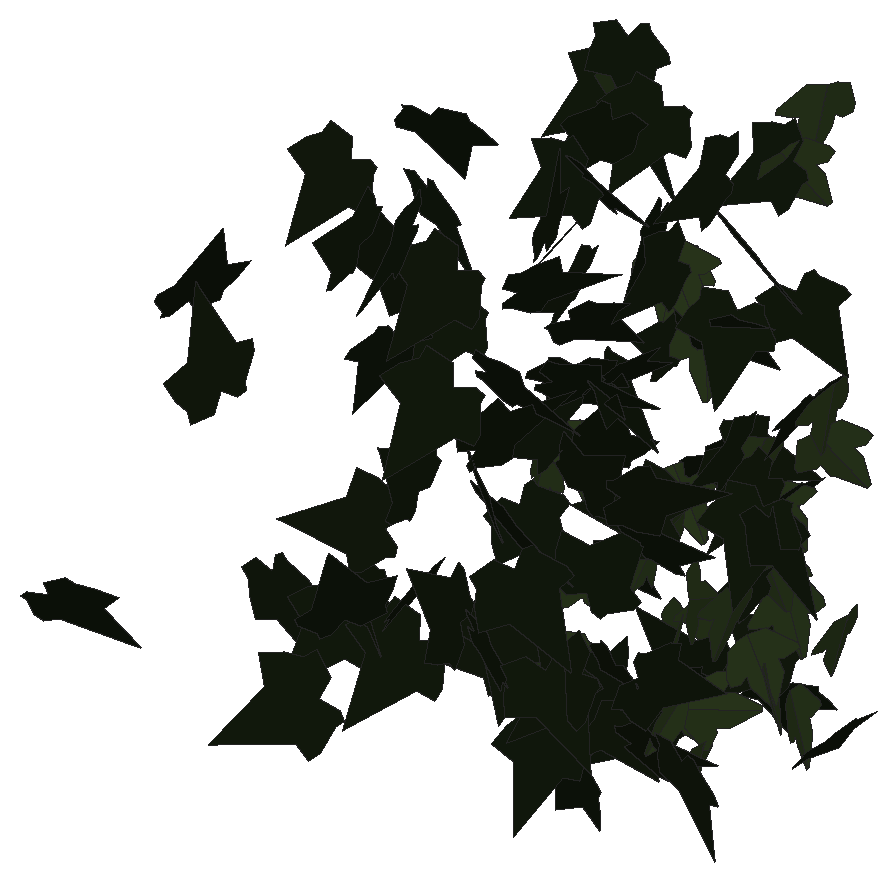
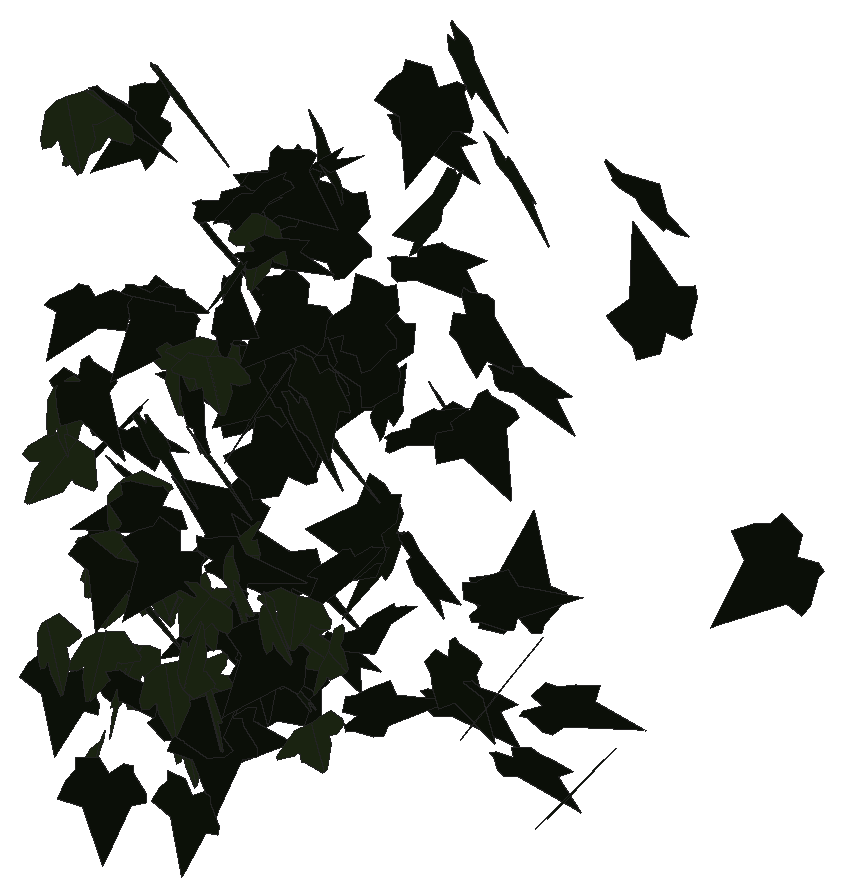
# SketchUp Ruby script. Lengths in inches.
U = 1.inch
M = Sketchup.active_model
def pt(a) = Geom::Point3d.new(a.map { |v| v * U })
def face(e, loops, mat)
  f = e.add_face(loops[0].map { |a| pt(a) })
  loops[1..].each { |l| e.add_face(l.map { |a| pt(a) }).erase! }
  f.material = f.back_material = mat if mat
  f
end
# faces: each face lists its corners as indices into pts; further lists are holes
def faces(e, pts, list, mat = nil) = list.each { |f| face(e, (f[0].is_a?(Array) ? f : [f]).map { |l| l.map { |i| pts[i] } }, mat) }
# xy, xz, yz: faces in a plane at the given z, y or x. An outline is a flat list of corners, or four numbers for a rectangle; further outlines are holes
def ring(l) = l.size == 4 ? [[l[0], l[1]], [l[2], l[1]], [l[2], l[3]], [l[0], l[3]]] : l.each_slice(2).to_a
def flat(e, list, mat, &to3) = list.each { |f| face(e, (f[0].is_a?(Array) ? f : [f]).map { |l| ring(l).map { |u, v| to3.(u, v) } }, mat) }
def xy(e, z, list, mat = nil) = flat(e, list, mat) { |x, y| [x, y, z] }
def xz(e, y, list, mat = nil) = flat(e, list, mat) { |x, z| [x, y, z] }
def yz(e, x, list, mat = nil) = flat(e, list, mat) { |y, z| [x, y, z] }
def lines(e, pts, list) = list.each { |a, b| e.add_line(pt(pts[a]), pt(pts[b])) }
# prism: a flat outline (further loops are holes) pulled along v
def prism(e, loops, v, mat = nil)
  f = face(e, loops, mat); d = Geom::Vector3d.new(v.map { |x| x * U })
  f.pushpull(f.normal.samedirection?(d) ? d.length : -d.length)
end
def box(e, o, s, mat = nil) = prism(e, [[o, [o[0] + s[0], o[1], o[2]], [o[0] + s[0], o[1] + s[1], o[2]], [o[0], o[1] + s[1], o[2]]]], [0, 0, s[2]], mat)
def at(x, y, z, deg = 0) = Geom::Transformation.translation(pt([x, y, z])) * Geom::Transformation.rotation(ORIGIN, Z_AXIS, deg.degrees)
def axes(o, x, y, z) = Geom::Transformation.new([*x, 0, *y, 0, *z, 0, *pt(o).to_a, 1])
def part(name) = M.definitions.add(name)
# library, detail: a bought-in or finely detailed component or shape, given as its bounding box
def library(name, o, s) = part(name).tap { |d| box(d.entities, o, s) }
def detail(e, o, s) = box(e.add_group.entities, o, s)
def put(e, d, t, mat = nil) = e.add_instance(d, t).tap { |i| i.material = mat if mat }
def group(e, t, mat = nil) = e.add_group.tap { |g| g.transformation = t; g.material = mat if mat }.entities
root = M.entities
M.materials.add("efeu1").color = [18, 25, 13]
M.materials.add("efeu2").color = [43, 57, 29]
c1 = part("ivyleaf_9")
p = [[1.54,2.16,1.25],[1.36,2.04,1.19],[-0.21,0.99,0.68],[-0.71,1.11,0.82],[-0.85,0.86,0.67],[-0.8,0.17,0.21],
  [-0.9,-0.01,0.1],[-0.67,-0.16,-0.02],[-0.08,-0.08,-0.05],[-0.03,-0.6,-0.4],[0.65,-0.88,-0.66],[0.83,-0.6,-0.49],
  [1.29,-0.42,-0.43],[1.8125,-0.07,-0.26],[1.21,0.44,0.15]]
faces(c1.entities,p,[[0,1,2,3,4,5,6,7,8,9,10,11,12,13,14]],"efeu1")
c2 = part("ivyleaf_10")
p = [[0,0.5,-0.03],[-0.0625,2.02,-0.43],[-0.19,2.01,-0.46],[-0.54,1.05,-0.29],[-0.52,0.625,-0.18],[-0.83,0.76,-0.28],
  [-1.16,0.64,-0.33],[-1.15,0.33,-0.24],[-0.77,-0.39,0.02],[-0.3,-0.51,0.16],[0.04,-0.48,0.23],[-0.02,2.01,-0.4375],
  [-0.06,2.01,-0.43],[0.04,-0.49,0.23],[0.67,-0.49,0.14],[1.38,0.36,-0.2],[1.375,0.51,-0.24],[0.81,0.65,-0.19],
  [0.62,0.59,-0.15],[0.6,1.09,-0.28],[0.5,1.23,-0.31]]
faces(c2.entities,p,[[0,1,2,3,4,5,6,7,8,9,10],[11,12,0,13,14,15,16,17,18,19,20]],"efeu2")
put(root,c1,axes([487.93,108.94,283.27],[1.28047,0.4773,0.27345],[0.2614,0.10282,-1.3292],[-0.52728,1.21006,0.00509]))
put(root,c1,axes([488.25,120.74,279.03],[0.66531,-1.07107,-0.28603],[-0.01199,0.30882,-1.27663],[1.19422,0.5998,0.14653]))
put(root,c1,axes([490.58,121.86,295.7],[-1.24756,-0.33673,-0.124],[0.12614,0.02537,-1.25133],[0.36459,-1.16101,0.00862]))
put(root,c1,axes([490.5,113.3,294.06],[0.7519,0.9623,0.59354],[-0.36171,-0.4621,1.23525],[1.1529,-0.77257,0.00046]))
put(root,c1,axes([491.55,120.59,278.68],[-1.20578,-0.36706,0.02195],[-0.02114,-0.00803,-1.22226],[0.39652,-1.11663,0.00157]))
put(root,c1,axes([493.79,116.03,278.13],[-1.09165,-0.45472,0.71253],[-0.6746,-0.28149,-1.15269],[0.57758,-1.18821,0.0004]))
put(root,c1,axes([494.18,119.21,283.68],[-0.63666,-0.11353,1.04614],[-1.04545,-0.27731,-0.62254],[0.31983,-1.13246,0.04757]))
put(root,c1,axes([493.28,120.4,280.03],[0.56041,-1.01215,-0.61379],[0.28817,-0.52643,1.18291],[-1.23214,-0.58348,-0.00251]))
put(root,c1,axes([495.48,118.52,295.01],[-0.3234,0.18269,-1.25426],[-1.25926,-0.40761,0.23687],[-0.38692,1.17388,0.27745]))
put(root,c1,axes([494.85,119.17,291.41],[-0.01545,0.87558,-0.83789],[0.05178,-0.80465,-0.91033],[-1.28399,-0.04299,-0.02663]))
put(root,c1,axes([495.12,120.08,281.33],[-0.61436,0.86217,-0.53743],[0.23859,-0.47202,-1.07194],[-1.05905,-0.60649,0.07027]))
put(root,c1,axes([495.47,119.46,279.48],[-1.26791,-0.58004,0.05064],[-0.04795,-0.02007,-1.36184],[0.62682,-1.17482,-0.00174]))
put(root,c1,axes([494.96,116.24,281.73],[0.81621,0.50536,0.90532],[-0.76893,-0.50108,0.94538],[0.76843,-1.03819,-0.01561]))
put(root,c1,axes([496.25,107.69,295.03],[-1.35018,0.22059,-0.35895],[-0.37798,0.00073,1.31888],[0.22987,1.29694,0.06031]))
put(root,c1,axes([495.56,121.73,291.72],[-0.62945,-0.9519,0.32133],[-0.13909,-0.28323,-1.16017],[1.07186,-0.59576,0.03815]))
put(root,c2,axes([496,126.03,283.95],[-0.05585,0.76733,-0.76603],[-0.02611,-0.7381,-0.79792],[-1.14844,-0.02054,0.0554]))
put(root,c1,axes([497.65,113.55,298.5625],[-0.71399,0.92904,0.58294],[-0.32129,0.47602,-1.18544],[-1.12693,-0.72432,-0.03136]))
put(root,c1,axes([497.79,121.96,278.97],[-0.63673,-0.23437,0.99321],[-0.89864,-0.4745,-0.65533],[0.56597,-1.01709,0.07686]))
put(root,c1,axes([498,124.14,294.07],[-0.22195,1.05914,0.2908],[-0.07545,0.27124,-1.12192],[-1.18065,-0.21644,0.01703]))
put(root,c1,axes([498.6,115.63,288.34],[-0.44952,0.70387,0.94859],[-0.52802,0.77025,-0.8502],[-1.1267,-0.6418,0.01998]))
put(root,c2,axes([498.64,126.44,284.82],[-0.33345,0.24798,1.01054],[-1.02586,0.25368,-0.38123],[-0.34727,-0.98748,0.15583]))
put(root,c2,axes([497.55,125.99,285.46],[1.05762,0.34197,0.24255],[0.23343,0.08843,-1.07869],[-0.38126,1.00277,0.01241]))
put(root,c1,axes([498.62,124.46,292.66],[-0.76152,0.84642,0.12193],[-0.0679,0.1002,-1.14559],[-0.92036,-0.70774,-0.01637]))
put(root,c1,axes([497.37,117.9,298.62],[0.82838,-0.99614,0.21737],[0.14057,-0.16356,-1.30751],[1.09023,0.77798,0.00343]))
put(root,c1,axes([499.32,116.99,282.75],[-0.77408,0.11861,-1.07409],[-1.12199,-0.03607,0.74551],[0.04086,1.2566,0.12278]))
put(root,c1,axes([498.6,116.57,302.58],[1.06494,0.63385,-0.42408],[-0.39134,-0.1901,-1.21858],[-0.71374,1.04997,0.03539]))
put(root,c1,axes([499.18,126.26,299.9],[-0.97309,-0.47861,0.43077],[-0.36109,-0.25196,-1.05916],[0.58044,-0.95912,0.06328]))
put(root,c2,axes([498.79,123.53,278.63],[0.45745,0.95813,-0.33869],[-0.12878,-0.30333,-1.0894],[-1.08531,0.43984,-0.0135]))
put(root,c1,axes([498.61,121.46,285.01],[0.27665,-0.81103,-0.82368],[-0.03201,0.8069,-0.86931],[1.22386,0.20444,0.16346]))
put(root,c2,axes([499.94,123.3,282.11],[0.43654,0.59015,-0.87113],[-0.85601,-0.39058,-0.68397],[-0.70132,0.84407,0.29258]))
put(root,c1,axes([499.2,120.26,281.35],[-0.29354,-1.2558,0.10971],[0.04408,-0.11663,-1.3346],[1.36033,-0.26721,0.06692]))
put(root,c2,axes([499.65,125.52,300.19],[-1.17327,0.17833,-0.01914],[0.01141,-0.04912,-1.14391],[-0.19328,-1.08541,0.04862]))
put(root,c1,axes([498.58,120.01,285.47],[0.96236,-0.64468,0.71352],[0.61154,-0.38769,-1.14371],[0.81229,1.05565,0.01571]))
put(root,c1,axes([499.54,124.47,282.3125],[1.08086,0.50793,0.05554],[0.04126,0.0427,-1.167],[-0.55004,1.00131,0.02159]))
put(root,c1,axes([499.7,125.96,301.93],[-0.00715,-1.08085,-0.28112],[-0.01614,0.27037,-1.12398],[1.20316,-0.0028,-0.01675]))
put(root,c1,axes([501.16,120.59,289.69],[-1.08825,0.75622,0.20973],[-0.21335,0.07236,-1.30875],[-0.81789,-1.02507,0.06234]))
put(root,c1,axes([499.99,126,299.13],[0.71012,-0.86332,-0.21957],[-0.17465,0.14202,-1.12777],[0.94384,0.67582,-0.04349]))
put(root,c2,axes([500.81,128.3,282.34],[-0.99681,0.45304,-0.10562],[-0.09466,0.05192,1.06926],[0.49241,0.92709,-0.00827]))
put(root,c1,axes([501.09,114.36,293.66],[-1.1174,-0.74824,0.09783],[-0.09095,-0.04406,-1.32784],[0.80937,-1.03797,-0.01416]))
put(root,c1,axes([501.63,126.28,290.56],[-0.6962,0.71839,0.51384],[-0.36076,0.36408,-1.00381],[-0.8698,-0.72602,0.00506]))
put(root,c1,axes([501.32,120.99,291.74],[0.48216,0.89736,-0.57571],[-0.36034,-0.45002,-1.03853],[-1.0802,0.55067,0.08946]))
put(root,c1,axes([501.34,127.53,276.62],[0.05973,1.00849,0.27515],[0.00127,0.26488,-1.05032],[-1.12602,0.05379,0.01341]))
put(root,c1,axes([501.43,111.7,301.33],[-1.07069,0.64043,-0.56187],[0.49905,-0.28027,-1.22737],[-0.75485,-1.09369,-0.01448]))
put(root,c1,axes([501.48,122.65,300.73],[-0.16617,0.42284,-1.15158],[0.11729,-1.10686,-0.45527],[-1.27472,-0.15696,0.10823]))
put(root,c1,axes([500.78,116.33,282.95],[1.11311,-0.44226,-0.57466],[-0.51259,0.29221,-1.16392],[0.56703,1.13234,0.07591]))
put(root,c1,axes([500.73,116.72,288.3],[-0.11743,-0.19889,1.22297],[0.35877,-1.13913,-0.16843],[1.23707,0.31149,0.16494]))
put(root,c1,axes([500.75,116.47,290.38],[0.41054,0.09554,1.27946],[0.993,0.83661,-0.36303],[-0.8888,0.97882,0.1854]))
put(root,c1,axes([500.34,117.6,292.59],[1.09496,-0.2857,0.58591],[0.58305,-0.16126,-1.09544],[0.35422,1.1486,-0.00806]))
put(root,c1,axes([501.75,113.72,298.82],[-1.29927,-0.40781,-0.08882],[0.09054,0.0187,-1.32104],[0.44079,-1.20591,0.00956]))
put(root,c1,axes([502.3,121.1,278.99],[-0.19234,0.78394,0.95988],[-0.66464,0.74484,-0.78146],[-1.12635,-0.57339,0.29721]))
put(root,c1,axes([501.76,120.65,299.54],[-0.62074,-0.59858,0.79763],[-0.32321,-0.73882,-0.83294],[0.99977,-0.6105,0.22595]))
put(root,c1,axes([502.66,124.33,284.79],[-0.76552,0.11117,0.89511],[-0.92454,0.09292,-0.74568],[-0.15391,-1.11111,0.0272]))
put(root,c1,axes([501.95,124.92,300.42],[-0.86795,-0.80642,0.09014],[-0.06237,-0.06482,-1.18403],[0.87373,-0.80572,0.00503]))
put(root,c1,axes([501.33,121.95,287.95],[1.12729,0.53463,0.35878],[-0.35836,-0.10816,1.21842],[0.58634,-1.09399,0.05487]))
put(root,c2,axes([501.18,126.81,284.625],[0.92731,0.25344,0.61982],[0.61929,0.16252,-0.93104],[-0.32511,1.03248,-0.00559]))
put(root,c2,axes([501.67,125.95,294.04],[1.1014,0.3935,-0.06883],[-0.05703,-0.04694,-1.13653],[-0.42716,1.02088,-0.02573]))
put(root,c1,axes([501.01,120.42,291.29],[1.04245,0.17584,0.70002],[0.69592,0.20798,-1.01749],[-0.28323,1.15822,0.07643]))
put(root,c2,axes([501.86,126.06,283.59],[-0.27404,0.07877,-1.10356],[-0.06938,-1.09002,-0.06817],[-1.14706,0.04711,0.26777]))
put(root,c1,axes([502.21,124.88,278.04],[0.47069,0.90796,-0.34427],[-0.21132,-0.27271,-1.04584],[-1.02212,0.4745,0.05769]))
put(root,c1,axes([501.86,124.9,296.1],[-0.37104,0.20867,-1.1142],[0.85439,-0.72621,-0.41094],[-0.81214,-0.85932,0.07672]))
put(root,c2,axes([502.09,125.56,279.9375],[0.73965,-0.77122,-0.18777],[-0.10942,0.15143,-1.07237],[0.84841,0.69188,0.0254]))
put(root,c2,axes([502.15,124.03,283.66],[0.87236,-0.64345,-0.2581],[-0.21431,0.1492,-1.07399],[0.71333,0.83173,-0.00702]))
put(root,c1,axes([502.36,126.11,291.32],[0.38643,-0.24422,1.04412],[-0.31924,0.99386,0.361],[-1.06926,-0.38499,0.26957]))
put(root,c2,axes([501.83,124.34,285.1875],[-0.18245,-0.42391,1.02305],[0.45538,-0.94178,-0.34677],[1.06345,0.33055,0.32401]))
put(root,c1,axes([501.58,121.44,282.88],[-0.56165,0.1282,1.07476],[1.08545,-0.24053,0.55703],[0.29435,1.13161,-0.00335]))
put(root,c1,axes([501.83,120.33,294.07],[0.85819,0.74328,0.39027],[0.27186,0.28,-1.13114],[-0.85717,0.83297,0.03198]))
put(root,c1,axes([501.51,117.84,296.19],[0.72829,0.28454,0.97717],[0.80908,0.58756,-0.74422],[-0.68524,0.99616,0.15985]))
put(root,c1,axes([502.55,117.82,298.74],[0.25955,0.18739,1.17934],[-0.16147,1.15375,-0.16533],[-1.23076,-0.11185,0.27039]))
put(root,c1,axes([501.91,122.07,291.21],[0.73433,-0.68648,-0.64928],[-0.40161,0.50751,-1.00158],[0.91815,0.77104,0.08118]))
put(root,c1,axes([501.38,121.33,299.13],[0.63158,-0.5806,0.79494],[0.71759,-0.40109,-0.84552],[0.74814,0.87485,0.13992]))
put(root,c1,axes([502.94,125.85,277.94],[0.38619,-0.01669,1.08091],[-1.10846,0.16839,0.37005],[-0.17779,-1.08615,0.04076]))
put(root,c1,axes([502.55,124.13,277.1],[-0.04179,-0.26975,-1.11152],[0.28744,-1.04007,0.26299],[-1.15525,-0.24902,0.10564]))
put(root,c1,axes([502.32,121.58,291.38],[0.63093,0.72009,0.68314],[0.2286,0.65382,-0.9412],[-1.02754,0.58761,0.21008]))
put(root,c1,axes([502.52,118.14,278.81],[-1.12746,-0.4363,-0.48137],[0.51287,0.05723,-1.17001],[0.45704,-1.14052,0.12544]))
put(root,c1,axes([502.05,121.56,278.27],[-0.03804,-0.55808,-0.97336],[0.17425,0.92342,-0.57897],[1.16389,-0.15649,0.05487]))
put(root,c2,axes([502.125,125.28,294.22],[0.68518,0.81465,0.4026],[0.28504,0.2849,-1.07336],[-0.93147,0.68643,-0.0323]))
put(root,c1,axes([502.91,121.24,280.33],[0.71311,0.11141,-0.93054],[-0.95771,-0.1205,-0.69618],[-0.17626,1.10546,0.0179]))
put(root,c1,axes([503.28,118.62,277.74],[0.57218,0.07615,-1.17075],[-1.20371,-0.15818,-0.55665],[-0.1896,1.23406,0.00089]))
put(root,c1,axes([502.64,126.74,286.19],[0.80012,0.75551,0.2424],[0.16171,0.17956,-1.1003],[-0.83844,0.75561,0.0191]))
put(root,c1,axes([503.68,118.25,281.59],[-1.32583,0.18694,-0.04933],[0.05068,-0.00694,-1.29145],[-0.20203,-1.22852,-0.00021]))
put(root,c2,axes([503.22,126.55,280.57],[-0.55458,-0.9302,0.11552],[0.02497,-0.13921,-1.10131],[1.01144,-0.5066,0.09052]))
put(root,c1,axes([502.63,117.8,281.45],[0.10065,-1.16133,-0.42871],[0.45424,0.41855,-1.12744],[1.251,-0.05854,0.44387]))
put(root,c1,axes([502.77,119.69,288],[-0.30474,0.02546,1.15088],[0.82637,-0.82073,0.22254],[0.86385,0.79411,0.19311]))
put(root,c2,axes([504.26,123.17,278.59],[0.1781,0.64372,-0.88062],[-0.28625,-0.80497,-0.69011],[-1.11251,0.31017,0.03659]))
put(root,c1,axes([504.51,128.46,276.83],[0.62597,0.78464,-0.48189],[-0.41775,-0.27728,-0.99414],[-0.82059,0.73971,0.1385]))
put(root,c1,axes([503.35,121.76,277.2],[0.67191,0.38023,-0.85119],[0.77747,0.39043,0.75773],[0.5878,-0.95105,-0.02923]))
put(root,c1,axes([503.375,122.19,285],[0.35737,-0.41347,1.02572],[0.98992,-0.42222,-0.50391],[0.59503,0.95076,0.22228]))
put(root,c1,axes([504.99,121.9,296.79],[-1.16792,0.31848,-0.11473],[0.11074,-0.0423,-1.17236],[-0.34675,-1.0862,0.01201]))
put(root,c1,axes([504,114.4,287.4],[0.04431,-0.92423,-0.92716],[0.11494,0.89133,-0.95592],[1.38208,-0.0445,0.10923]))
put(root,c2,axes([504.32,124.28,292.48],[1.15954,0.00555,0.17754],[0.18162,0.15554,-1.10525],[-0.03223,1.07595,0.15886]))
put(root,c2,axes([504.77,123.56,276.6],[0.13233,-1.0526,0.01035],[0.00619,-0.00935,-1.10208],[1.13684,0.12258,0.0048]))
put(root,c1,axes([504.31,120.95,280.51],[0.17654,0.14581,-1.15367],[-0.09042,1.11953,0.14021],[1.20496,0.06264,0.17955]))
put(root,c1,axes([504.06,126.07,287.32],[0.40266,-0.08125,-1.07361],[0.35556,1.04956,0.03775],[1.06032,-0.3211,0.39505]))
put(root,c2,axes([504.9,122.98,282.99],[0.28504,-0.43932,-1.01289],[0.0195,1.0049,-0.46633],[1.15374,0.09155,0.25812]))
put(root,c1,axes([505.58,126.76,279.67],[-1.08801,-0.1908,0.1606],[-0.16871,-0.00482,-1.06604],[0.20448,-1.01917,-0.02503]))
put(root,c2,axes([505.24,126.24,287.55],[-0.39904,-0.98671,0.33539],[-0.01323,-0.33814,-1.09057],[1.12104,-0.35521,0.10651]))
put(root,c1,axes([505.48,126.86,285.17],[0.23931,1.02519,0.28621],[-0.00134,0.28138,-1.08911],[-1.1464,0.21368,0.06102]))
put(root,c1,axes([506.1,125.42,283.1875],[-0.90596,0.6776,0.16824],[-0.18879,0.02758,-1.12774],[-0.67216,-0.92103,0.09]))
put(root,c2,axes([504.91,123.53,278.44],[0.01734,-0.33008,-1.06308],[0.74353,0.7879,-0.25335],[0.89051,-0.65143,0.23223]))
put(root,c1,axes([506.17,123.95,288.94],[-0.88288,0.73626,-0.01154],[0.00909,-0.00723,-1.14417],[-0.7952,-0.81753,-0.00027]))
put(root,c2,axes([505.35,126.66,285.34],[0.63338,0.68092,0.64339],[0.30046,0.56805,-0.92451],[-0.94707,0.63559,0.13699]))
put(root,c2,axes([505.95,123.98,282.8],[-0.08131,-1.006,0.3883],[0.07211,-0.37795,-1.04509],[1.15665,-0.04716,0.09245]))
put(root,c2,axes([505.74,127.22,281.35],[-0.52626,-0.98427,-0.1825],[0.39017,-0.0118,-1.06145],[0.92188,-0.55688,0.34506]))
put(root,c2,axes([505.68,125.38,280.15],[0.56684,0.84903,0.38204],[0.09323,0.37556,-1.031],[-0.99474,0.51901,0.12108]))
put(root,c2,axes([505.87,127.51,277.05],[-0.2662,1.03026,-0.02855],[0.00781,-0.02649,-1.10171],[-1.11305,-0.24659,-0.0009]))
put(root,c1,axes([505.65,123.3,293.73],[1.02169,0.58885,0.15222],[0.11466,0.10629,-1.15834],[-0.6452,0.95135,0.03519]))
put(root,c1,axes([505.22,118.9,288.86],[0.47927,0.61608,-0.96379],[0.42365,0.84705,0.78099],[1.1247,-0.58159,0.11652]))
put(root,c2,axes([506.125,125.69,283.75],[-1.10358,-0.30049,-0.17545],[0.16277,0.08506,-1.10698],[0.33469,-1.03217,-0.04015]))
put(root,c2,axes([506.19,125.61,279.03],[-0.59656,0.87524,0.23249],[-0.17692,0.16062,-1.07503],[-0.95943,-0.57384,0.05368]))
put(root,c1,axes([506.59,124.87,287.38],[-1.14282,0.04162,-0.28699],[0.28922,-0.15305,-1.09198],[-0.08481,-1.08279,0.14332]))
put(root,c1,axes([506.28,123.63,294.43],[-0.83249,-0.72285,-0.39433],[0.35788,0.19949,-1.09613],[0.80565,-0.83555,0.07945]))
put(root,c1,axes([507.91,120.87,301.67],[-1.16317,0.6782,0.06532],[-0.05729,0.03364,-1.32367],[-0.73336,-1.07831,-0.00021]))
put(root,c1,axes([508.23,125.45,290.95],[-0.48046,0.93746,-0.52932],[0.10725,-0.53508,-1.045],[-1.07122,-0.47404,0.13279]))
put(root,c1,axes([507.44,125.67,294.7],[-0.11833,-0.67003,-0.92597],[0.1939,0.87235,-0.70572],[1.18773,-0.20917,0.02296]))
put(root,c2,axes([508.02,127.39,281.09],[0.06339,-1.06473,-0.02584],[-0.03838,0.02291,-1.10842],[1.14958,0.05947,-0.03558]))
put(root,c2,axes([508.14,126.19,302.54],[-0.51166,-1.07479,0.19416],[0.02017,-0.22367,-1.18501],[1.092,-0.49947,0.11286]))
put(root,c2,axes([507.83,126.75,288.57],[-0.81879,-0.54362,-0.64582],[0.57249,0.3036,-0.98138],[0.62037,-0.99766,0.05326]))
put(root,c2,axes([508.18,126.5,290.6],[0.01481,-1.17512,0.06251],[0.08506,-0.06129,-1.17219],[1.1737,0.01927,0.08416]))
put(root,c1,axes([508.89,123.33,301.49],[-1.16718,0.14608,0.27419],[-0.27223,0.03276,-1.17629],[-0.14971,-1.19851,0.00126]))
put(root,c1,axes([508.06,122.83,287.65],[-0.94547,-0.75402,-0.38621],[0.47728,0.04317,-1.17464],[0.77215,-0.94996,0.25316]))
put(root,c1,axes([509.22,125.02,277.95],[0.18021,1.08455,0.29208],[-0.10254,0.29661,-1.13259],[-1.2056,0.13689,0.13999]))
put(root,c2,axes([508.7,123.62,301.35],[-0.71728,-0.73165,-0.63379],[0.50272,0.39253,-1.02209],[0.8272,-0.87298,0.0716]))
put(root,c1,axes([508.41,120.73,299.85],[1.25605,-0.45755,-0.02533],[-0.02417,0.00964,-1.29976],[0.49426,1.16322,0.00081]))
put(root,c1,axes([508.48,118.02,279.84],[0.54099,-1.09533,0.45129],[0.2161,-0.38559,-1.25244],[1.25393,0.53902,0.02114]))
put(root,c1,axes([508.6875,122.6,287.49],[0.56502,-1.02328,-0.34226],[-0.07177,0.33452,-1.1916],[1.15867,0.51972,0.09309]))
